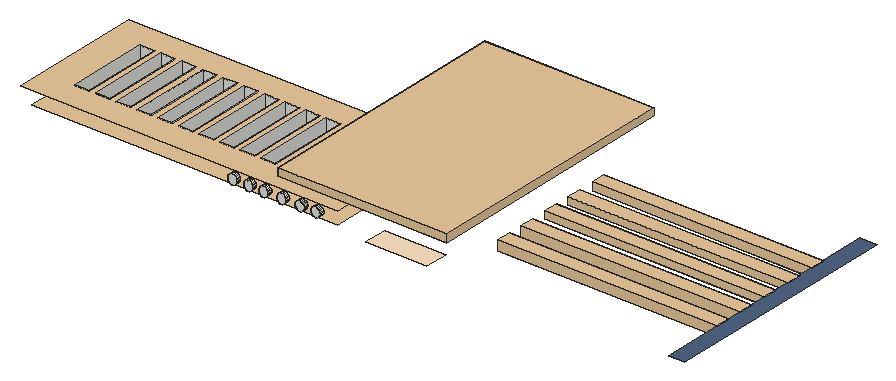
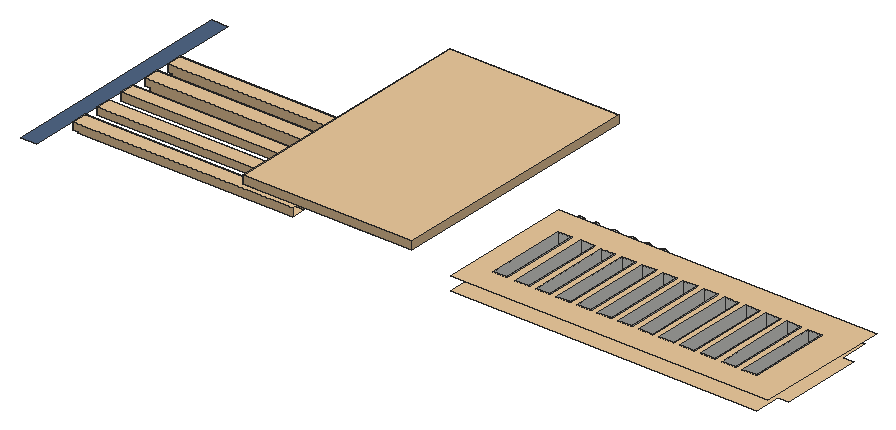
# SketchUp Ruby script. Lengths in inches.
U = 1.inch
M = Sketchup.active_model
def pt(a) = Geom::Point3d.new(a.map { |v| v * U })
def face(e, loops, mat)
  f = e.add_face(loops[0].map { |a| pt(a) })
  loops[1..].each { |l| e.add_face(l.map { |a| pt(a) }).erase! }
  f.material = f.back_material = mat if mat
  f
end
# faces: each face lists its corners as indices into pts; further lists are holes
def faces(e, pts, list, mat = nil) = list.each { |f| face(e, (f[0].is_a?(Array) ? f : [f]).map { |l| l.map { |i| pts[i] } }, mat) }
# xy, xz, yz: faces in a plane at the given z, y or x. An outline is a flat list of corners, or four numbers for a rectangle; further outlines are holes
def ring(l) = l.size == 4 ? [[l[0], l[1]], [l[2], l[1]], [l[2], l[3]], [l[0], l[3]]] : l.each_slice(2).to_a
def flat(e, list, mat, &to3) = list.each { |f| face(e, (f[0].is_a?(Array) ? f : [f]).map { |l| ring(l).map { |u, v| to3.(u, v) } }, mat) }
def xy(e, z, list, mat = nil) = flat(e, list, mat) { |x, y| [x, y, z] }
def xz(e, y, list, mat = nil) = flat(e, list, mat) { |x, z| [x, y, z] }
def yz(e, x, list, mat = nil) = flat(e, list, mat) { |y, z| [x, y, z] }
def lines(e, pts, list) = list.each { |a, b| e.add_line(pt(pts[a]), pt(pts[b])) }
# prism: a flat outline (further loops are holes) pulled along v
def prism(e, loops, v, mat = nil)
  f = face(e, loops, mat); d = Geom::Vector3d.new(v.map { |x| x * U })
  f.pushpull(f.normal.samedirection?(d) ? d.length : -d.length)
end
def box(e, o, s, mat = nil) = prism(e, [[o, [o[0] + s[0], o[1], o[2]], [o[0] + s[0], o[1] + s[1], o[2]], [o[0], o[1] + s[1], o[2]]]], [0, 0, s[2]], mat)
def at(x, y, z, deg = 0) = Geom::Transformation.translation(pt([x, y, z])) * Geom::Transformation.rotation(ORIGIN, Z_AXIS, deg.degrees)
def axes(o, x, y, z) = Geom::Transformation.new([*x, 0, *y, 0, *z, 0, *pt(o).to_a, 1])
def part(name) = M.definitions.add(name)
# library, detail: a bought-in or finely detailed component or shape, given as its bounding box
def library(name, o, s) = part(name).tap { |d| box(d.entities, o, s) }
def detail(e, o, s) = box(e.add_group.entities, o, s)
def put(e, d, t, mat = nil) = e.add_instance(d, t).tap { |i| i.material = mat if mat }
def group(e, t, mat = nil) = e.add_group.tap { |g| g.transformation = t; g.material = mat if mat }.entities
root = M.entities
M.materials.add("[0012_Bisque]").color = [255, 228, 196]
M.materials.add("[0035_Tan]").color = [234, 201, 156]
M.materials.add("[Leather Blue]").color = [80, 102, 132]
prism(root,[[[493.92,509.25,1252],[495.54,509.25,1253.24],[497.43,509.25,1254.02],[499.45,509.25,1254.29],[501.47,509.25,1254.02],[503.35,509.25,1253.24],[504.97,509.25,1252],[506.21,509.25,1250.38],[506.99,509.25,1248.5],[507.26,509.25,1246.48],[506.99,509.25,1244.45],[506.21,509.25,1242.57],[504.97,509.25,1240.95],[503.35,509.25,1239.71],[501.47,509.25,1238.93],[499.45,509.25,1238.66],[497.43,509.25,1238.93],[495.54,509.25,1239.71],[493.92,509.25,1240.95],[492.68,509.25,1242.57],[491.9,509.25,1244.45],[491.63,509.25,1246.48],[491.9,509.25,1248.5],[492.68,509.25,1250.38]]],[0,-6.75,0])
prism(root,[[[355.92,509.25,1252],[357.54,509.25,1253.24],[359.43,509.25,1254.02],[361.45,509.25,1254.29],[363.47,509.25,1254.02],[365.35,509.25,1253.24],[366.97,509.25,1252],[368.21,509.25,1250.38],[368.99,509.25,1248.5],[369.26,509.25,1246.48],[368.99,509.25,1244.45],[368.21,509.25,1242.57],[366.97,509.25,1240.95],[365.35,509.25,1239.71],[363.47,509.25,1238.93],[361.45,509.25,1238.66],[359.43,509.25,1238.93],[357.54,509.25,1239.71],[355.92,509.25,1240.95],[354.68,509.25,1242.57],[353.9,509.25,1244.45],[353.63,509.25,1246.48],[353.9,509.25,1248.5],[354.68,509.25,1250.38]]],[0,-6.75,0])
prism(root,[[[467.74,509.25,1252],[469.35,509.25,1253.24],[471.24,509.25,1254.02],[473.26,509.25,1254.29],[475.28,509.25,1254.02],[477.17,509.25,1253.24],[478.78,509.25,1252],[480.03,509.25,1250.38],[480.81,509.25,1248.5],[481.07,509.25,1246.48],[480.81,509.25,1244.45],[480.03,509.25,1242.57],[478.78,509.25,1240.95],[477.17,509.25,1239.71],[475.28,509.25,1238.93],[473.26,509.25,1238.66],[471.24,509.25,1238.93],[469.35,509.25,1239.71],[467.74,509.25,1240.95],[466.49,509.25,1242.57],[465.71,509.25,1244.45],[465.45,509.25,1246.48],[465.71,509.25,1248.5],[466.49,509.25,1250.38]]],[0,-6.75,0])
prism(root,[[[382.49,509.25,1252],[384.1,509.25,1253.24],[385.99,509.25,1254.02],[388.01,509.25,1254.29],[390.03,509.25,1254.02],[391.92,509.25,1253.24],[393.53,509.25,1252],[394.78,509.25,1250.38],[395.56,509.25,1248.5],[395.82,509.25,1246.48],[395.56,509.25,1244.45],[394.78,509.25,1242.57],[393.53,509.25,1240.95],[391.92,509.25,1239.71],[390.03,509.25,1238.93],[388.01,509.25,1238.66],[385.99,509.25,1238.93],[384.1,509.25,1239.71],[382.49,509.25,1240.95],[381.24,509.25,1242.57],[380.46,509.25,1244.45],[380.2,509.25,1246.48],[380.46,509.25,1248.5],[381.24,509.25,1250.38]]],[0,-6.75,0])
prism(root,[[[437.36,509.25,1252],[438.98,509.25,1253.24],[440.86,509.25,1254.02],[442.88,509.25,1254.29],[444.91,509.25,1254.02],[446.79,509.25,1253.24],[448.41,509.25,1252],[449.65,509.25,1250.38],[450.43,509.25,1248.5],[450.7,509.25,1246.48],[450.43,509.25,1244.45],[449.65,509.25,1242.57],[448.41,509.25,1240.95],[446.79,509.25,1239.71],[444.91,509.25,1238.93],[442.88,509.25,1238.66],[440.86,509.25,1238.93],[438.98,509.25,1239.71],[437.36,509.25,1240.95],[436.12,509.25,1242.57],[435.34,509.25,1244.45],[435.07,509.25,1246.48],[435.34,509.25,1248.5],[436.12,509.25,1250.38]]],[0,-6.75,0])
prism(root,[[[407.67,509.25,1252],[409.29,509.25,1253.24],[411.18,509.25,1254.02],[413.2,509.25,1254.29],[415.22,509.25,1254.02],[417.1,509.25,1253.24],[418.72,509.25,1252],[419.96,509.25,1250.38],[420.74,509.25,1248.5],[421.01,509.25,1246.48],[420.74,509.25,1244.45],[419.96,509.25,1242.57],[418.72,509.25,1240.95],[417.1,509.25,1239.71],[415.22,509.25,1238.93],[413.2,509.25,1238.66],[411.18,509.25,1238.93],[409.29,509.25,1239.71],[407.67,509.25,1240.95],[406.43,509.25,1242.57],[405.65,509.25,1244.45],[405.38,509.25,1246.48],[405.65,509.25,1248.5],[406.43,509.25,1250.38]]],[0,-6.75,0])
xy(root,1235.23,[[[23.8,509.25,23.8,555.46,5.5,555.46,5.5,690.86,23.8,690.86,23.8,733.33,529.97,733.33,529.97,509.25],[92.76,555.46,116.39,690.86],[195.69,555.46,219.33,690.86],[58.44,555.46,82.08,690.86],[127.07,555.46,150.71,690.86],[161.38,555.46,185.02,690.86],[230.01,555.46,253.64,690.86],[264.32,555.46,287.96,690.86],[298.32,555.46,321.96,690.86],[332.32,555.46,355.96,690.86],[400.32,555.46,423.96,690.86],[471.51,555.46,495.14,690.86],[366.32,555.46,389.96,690.86],[434.32,555.46,457.96,690.86]]],"[0035_Tan]")
xy(root,1256.625,[[[5.5,509.25,529.97,733.33],[92.76,555.46,116.39,690.86],[195.69,555.46,219.33,690.86],[58.44,555.46,82.08,690.86],[127.07,555.46,150.71,690.86],[161.38,555.46,185.02,690.86],[230.01,555.46,253.64,690.86],[264.32,555.46,287.96,690.86],[298.32,555.46,321.96,690.86],[332.32,555.46,355.96,690.86],[400.32,555.46,423.96,690.86],[471.51,555.46,495.14,690.86],[366.32,555.46,389.96,690.86],[434.32,555.46,457.96,690.86]]],"[0035_Tan]")
xy(root,1266.48,[[771.27,586.45,1126.57,611.06]],"[0035_Tan]")
xy(root,1268.97,[[771.27,539.27,1126.57,563.87]],"[0035_Tan]")
xy(root,1271.04,[[771.27,734.95,1126.57,759.56]],"[0035_Tan]")
xy(root,1271.79,[[1126.57,539.27,1134.07,563.87]])
xy(root,1272.79,[[1126.57,586.45,1134.07,611.06],[771.27,636.14,1126.57,638.15],[1126.57,636.14,1134.07,638.15],[1126.57,638.15,1134.07,660.75],[1126.57,685.02,1134.07,709.62],
  [1126.57,734.95,1134.07,759.56]])
xy(root,1272.79,[[771.27,638.15,1126.57,660.75],[771.27,685.02,1126.57,709.62]],"[0035_Tan]")
xy(root,1276.62,[[633.21,439.49,733.59,478.61]],"[0012_Bisque]")
xy(root,1284.8125,[[771.27,539.27,1134.07,563.87],[771.27,586.45,1134.07,611.06],[771.27,636.14,1134.07,660.75],[771.27,685.02,1134.07,709.62],[771.27,734.95,1134.07,759.56]],"[0035_Tan]")
xy(root,1284.8125,[[1134.07,439.49,1160.87,835.03]],"[Leather Blue]")
xy(root,1345.9375,[[529.97,439.49,771.27,808.22],[529.97,808.22,615.34,835.03],[615.34,808.22,633.21,835.03],[633.21,808.22,748.59,835.03],[748.59,808.22,771.27,835.03],
  [771.27,808.22,792.33,835.03]])
xy(root,1345.9375,[[512.53,407.8,512.53,439.49,771.27,439.49,771.27,808.22,792.33,808.22,792.33,407.8],[512.53,439.49,529.97,470.4375],[512.53,470.4375,529.97,835.03]],"[0035_Tan]")
xy(root,1358.6875,[[512.53,407.8,792.33,835.03]],"[0035_Tan]")
xz(root,407.8,[[512.53,1345.9375,792.33,1358.6875]],"[0035_Tan]")
xz(root,539.27,[[771.27,1268.97,1126.57,1268.97,1126.57,1271.79,1134.07,1271.79,1134.07,1284.8125,771.27,1284.8125]],"[0035_Tan]")
xz(root,555.46,[[58.44,1235.23,82.08,1256.625],[92.76,1235.23,116.39,1256.625],[127.07,1235.23,150.71,1256.625],[161.38,1235.23,185.02,1256.625],[195.69,1235.23,219.33,1256.625],
  [230.01,1235.23,253.64,1256.625],[264.32,1235.23,287.96,1256.625],[298.32,1235.23,321.96,1256.625],[332.32,1235.23,355.96,1256.625],[366.32,1235.23,389.96,1256.625],
  [400.32,1235.23,423.96,1256.625],[434.32,1235.23,457.96,1256.625],[471.51,1235.23,495.14,1256.625]])
xz(root,563.87,[[771.27,1268.97,771.27,1284.8125,1134.07,1284.8125,1134.07,1271.79,1126.57,1271.79,1126.57,1268.97]],"[0035_Tan]")
xz(root,586.45,[[771.27,1266.48,1126.57,1266.48,1126.57,1272.79,1134.07,1272.79,1134.07,1284.8125,771.27,1284.8125]],"[0035_Tan]")
xz(root,611.06,[[771.27,1266.48,771.27,1284.8125,1134.07,1284.8125,1134.07,1272.79,1126.57,1272.79,1126.57,1266.48]],"[0035_Tan]")
xz(root,636.14,[[771.27,1272.79,1134.07,1284.8125]],"[0035_Tan]")
xz(root,660.75,[[771.27,1272.79,1134.07,1284.8125]],"[0035_Tan]")
xz(root,685.02,[[771.27,1272.79,1134.07,1284.8125]],"[0035_Tan]")
xz(root,690.86,[[58.44,1235.23,82.08,1256.625],[92.76,1235.23,116.39,1256.625],[127.07,1235.23,150.71,1256.625],[161.38,1235.23,185.02,1256.625],[195.69,1235.23,219.33,1256.625],
  [230.01,1235.23,253.64,1256.625],[264.32,1235.23,287.96,1256.625],[298.32,1235.23,321.96,1256.625],[332.32,1235.23,355.96,1256.625],[366.32,1235.23,389.96,1256.625],
  [400.32,1235.23,423.96,1256.625],[434.32,1235.23,457.96,1256.625],[471.51,1235.23,495.14,1256.625]])
xz(root,709.62,[[771.27,1272.79,1134.07,1284.8125]],"[0035_Tan]")
xz(root,734.95,[[771.27,1271.04,1126.57,1271.04,1126.57,1272.79,1134.07,1272.79,1134.07,1284.8125,771.27,1284.8125]],"[0035_Tan]")
xz(root,759.56,[[771.27,1271.04,771.27,1284.8125,1134.07,1284.8125,1134.07,1272.79,1126.57,1272.79,1126.57,1271.04]],"[0035_Tan]")
xz(root,835.03,[[512.53,1345.9375,792.33,1358.6875]],"[0035_Tan]")
yz(root,58.44,[[555.46,1235.23,690.86,1256.625]])
yz(root,82.08,[[555.46,1235.23,690.86,1256.625]])
yz(root,92.76,[[555.46,1235.23,690.86,1256.625]])
yz(root,116.39,[[555.46,1235.23,690.86,1256.625]])
yz(root,127.07,[[555.46,1235.23,690.86,1256.625]])
yz(root,150.71,[[555.46,1235.23,690.86,1256.625]])
yz(root,161.38,[[555.46,1235.23,690.86,1256.625]])
yz(root,185.02,[[555.46,1235.23,690.86,1256.625]])
yz(root,195.69,[[555.46,1235.23,690.86,1256.625]])
yz(root,219.33,[[555.46,1235.23,690.86,1256.625]])
yz(root,230.01,[[555.46,1235.23,690.86,1256.625]])
yz(root,253.64,[[555.46,1235.23,690.86,1256.625]])
yz(root,264.32,[[555.46,1235.23,690.86,1256.625]])
yz(root,287.96,[[555.46,1235.23,690.86,1256.625]])
yz(root,298.32,[[555.46,1235.23,690.86,1256.625]])
yz(root,321.96,[[555.46,1235.23,690.86,1256.625]])
yz(root,332.32,[[555.46,1235.23,690.86,1256.625]])
yz(root,355.96,[[555.46,1235.23,690.86,1256.625]])
yz(root,366.32,[[555.46,1235.23,690.86,1256.625]])
yz(root,389.96,[[555.46,1235.23,690.86,1256.625]])
yz(root,400.32,[[555.46,1235.23,690.86,1256.625]])
yz(root,423.96,[[555.46,1235.23,690.86,1256.625]])
yz(root,434.32,[[555.46,1235.23,690.86,1256.625]])
yz(root,457.96,[[555.46,1235.23,690.86,1256.625]])
yz(root,471.51,[[555.46,1235.23,690.86,1256.625]])
yz(root,495.14,[[555.46,1235.23,690.86,1256.625]])
yz(root,512.53,[[407.8,1345.9375,835.03,1358.6875]],"[0035_Tan]")
yz(root,792.33,[[407.8,1345.9375,835.03,1358.6875]],"[0035_Tan]")
yz(root,1126.57,[[586.45,1266.48,611.06,1272.79],[539.27,1268.97,563.87,1271.79],[734.95,1271.04,759.56,1272.79]])
yz(root,1134.07,[[539.27,1271.79,563.87,1284.8125],[586.45,1272.79,611.06,1284.8125],[636.14,1272.79,660.75,1284.8125],[685.02,1272.79,709.62,1284.8125],[734.95,1272.79,759.56,1284.8125]])
